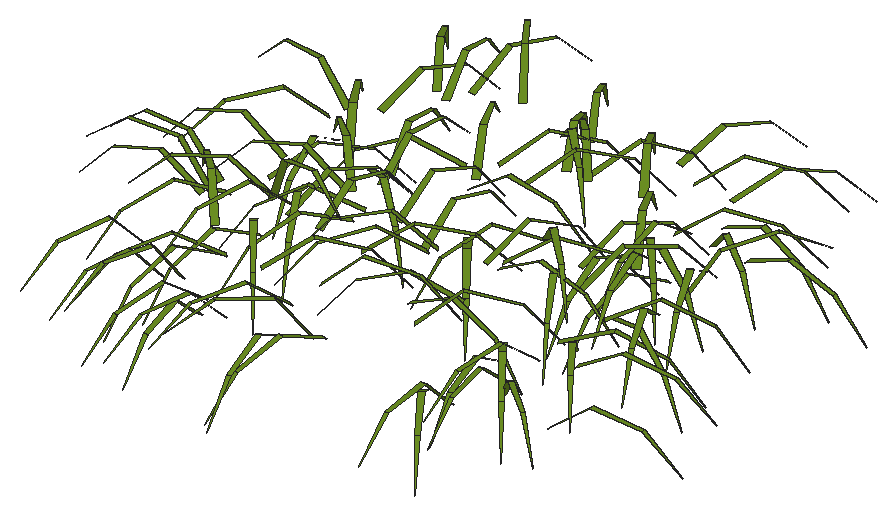
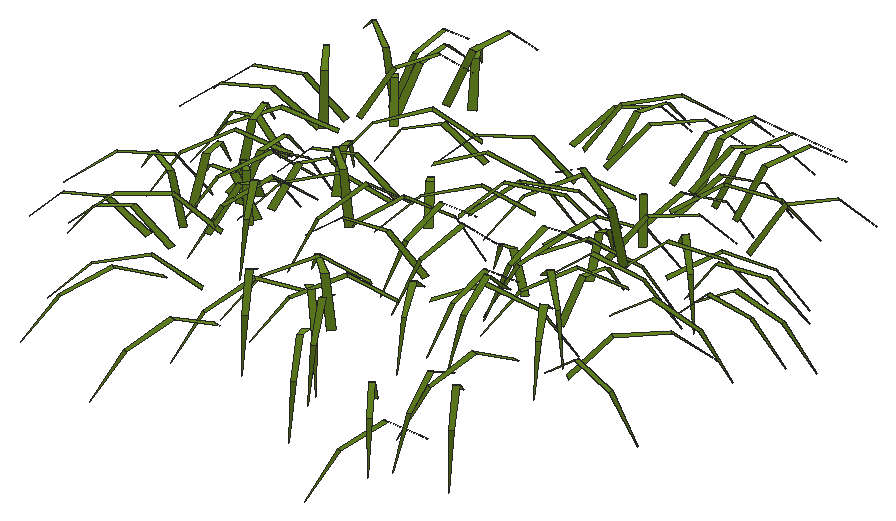
# SketchUp Ruby script. Lengths in inches.
U = 1.inch
M = Sketchup.active_model
def pt(a) = Geom::Point3d.new(a.map { |v| v * U })
def face(e, loops, mat)
  f = e.add_face(loops[0].map { |a| pt(a) })
  loops[1..].each { |l| e.add_face(l.map { |a| pt(a) }).erase! }
  f.material = f.back_material = mat if mat
  f
end
# faces: each face lists its corners as indices into pts; further lists are holes
def faces(e, pts, list, mat = nil) = list.each { |f| face(e, (f[0].is_a?(Array) ? f : [f]).map { |l| l.map { |i| pts[i] } }, mat) }
# xy, xz, yz: faces in a plane at the given z, y or x. An outline is a flat list of corners, or four numbers for a rectangle; further outlines are holes
def ring(l) = l.size == 4 ? [[l[0], l[1]], [l[2], l[1]], [l[2], l[3]], [l[0], l[3]]] : l.each_slice(2).to_a
def flat(e, list, mat, &to3) = list.each { |f| face(e, (f[0].is_a?(Array) ? f : [f]).map { |l| ring(l).map { |u, v| to3.(u, v) } }, mat) }
def xy(e, z, list, mat = nil) = flat(e, list, mat) { |x, y| [x, y, z] }
def xz(e, y, list, mat = nil) = flat(e, list, mat) { |x, z| [x, y, z] }
def yz(e, x, list, mat = nil) = flat(e, list, mat) { |y, z| [x, y, z] }
def lines(e, pts, list) = list.each { |a, b| e.add_line(pt(pts[a]), pt(pts[b])) }
# prism: a flat outline (further loops are holes) pulled along v
def prism(e, loops, v, mat = nil)
  f = face(e, loops, mat); d = Geom::Vector3d.new(v.map { |x| x * U })
  f.pushpull(f.normal.samedirection?(d) ? d.length : -d.length)
end
def box(e, o, s, mat = nil) = prism(e, [[o, [o[0] + s[0], o[1], o[2]], [o[0] + s[0], o[1] + s[1], o[2]], [o[0], o[1] + s[1], o[2]]]], [0, 0, s[2]], mat)
def at(x, y, z, deg = 0) = Geom::Transformation.translation(pt([x, y, z])) * Geom::Transformation.rotation(ORIGIN, Z_AXIS, deg.degrees)
def axes(o, x, y, z) = Geom::Transformation.new([*x, 0, *y, 0, *z, 0, *pt(o).to_a, 1])
def part(name) = M.definitions.add(name)
# library, detail: a bought-in or finely detailed component or shape, given as its bounding box
def library(name, o, s) = part(name).tap { |d| box(d.entities, o, s) }
def detail(e, o, s) = box(e.add_group.entities, o, s)
def put(e, d, t, mat = nil) = e.add_instance(d, t).tap { |i| i.material = mat if mat }
def group(e, t, mat = nil) = e.add_group.tap { |g| g.transformation = t; g.material = mat if mat }.entities
root = M.entities
M.materials.add("[0061_OliveDrab]").color = [107, 142, 35]
p = [[550.53,11.4,559.14],[550.39,11.51,559.14],[549.55,10.29,556.97],[556.85,12.2,559.2],[556.66,12.31,559.2],[556.06,10.94,557.04],
  [577.17,15.06,559.01],[577.09,14.89,559.01],[578.69,14.24,557.03],[571.92,16.4,559.27],[571.73,16.43,559.27],[571.6,15.04,557.05],
  [563.83,16.5,559.26],[563.68,16.61,559.26],[562.95,15.5,556.99],[576.57,16.09,559.07],[576.66,15.91,559.07],[578.05,16.67,556.97],
  [576.4,19.42,559.1875],[576.52,19.23,559.1875],[577.66,20.13,557],[579.22,11.04,558.77],[579.24,10.84,558.77],[581.21,11.15,557.05],
  [578.46,24.97,558.98],[578.45,24.76,558.98],[580.31,24.75,557.13],[572.51,4.17,559.14],[572.34,4.06,559.14],[573.47,2.63,557.24],
  [555.28,6.22,559.4],[555.09,6.27,559.4],[554.83,4.85,557.21],[555.6,8.46,559.36],[555.42,8.51,559.36],[555.14,7.1,557.16],
  [573.62,8.49,559.26],[573.46,8.375,559.26],[574.51,7.18,557.17],[558.04,13.51,559.35],[557.85,13.4,559.35],[558.68,12.14,557.2],
  [566.88,14.53,559.26],[566.7,14.39,559.26],[567.76,13.2,557.17],[554.87,14.97,559.34],[554.78,15.13,559.34],[553.5625,14.3,557.16],
  [555.24,34.98,558.98],[555.45,34.9375,558.98],[555.73,36.81,557.15],[563.09,3.13,559.2],[562.89,3.1,559.2],[563.24,1.35,557.28],
  [563.18,3.54,559.21],[562.98,3.57,559.21],[562.76,1.79,557.3],[558.66,10.34,559.48],[558.5,10.21,559.48],[559.46,9.16,557.26],
  [570.14,12.38,559.46],[570.13,12.17,559.46],[571.64,12.22,557.3125],[560.76,17.37,559.375],[560.62,17.2,559.375],[561.9,16.28,557.27],
  [576.31,25.49,559.35],[576.28,25.28,559.35],[577.93,25.13,557.31],[571.17,14.64,559.53],[571,14.54,559.53],[571.9,13.28,557.41],
  [566.61,30.04,559.53],[566.8,29.93,559.53],[567.41,31.3125,557.38],[574.57,10.62,557.51],[574.61,10.28,557.51],[576.66,10.53,559.12],
  [576.63,10.81,559.12],[547.04,15.13,559.45],[547.03,15.34,559.45],[545.24,15.2,557.54],[559.88,32.26,559.5],[560.05,32.36,559.5],
  [559.0625,33.74,557.48],[567.3,34.4375,559.32],[567.52,34.38,559.32],[567.85,36.24,557.49],[562.55,12.23,559.61],[562.48,12.43,559.61],
  [560.89,11.8,557.61],[555.53,21.01,559.63],[555.44,21.21,559.63],[553.98,20.42,557.59],[560.97,29.51,559.69],[561.16,29.62,559.69],
  [560.25,30.98,557.64],[572.37,32.6,559.48],[572.54,32.52,559.48],[573.27,34.2,557.6],[556.51,3.61,559.64],[556.32,3.66,559.64],
  [555.94,1.98,557.66],[553.4,7.4,559.76],[553.26,7.54,559.76],[552.16,6.32,557.71],[570.82,16.45,559.67],[570.6,16.42,559.67],
  [570.94,14.78,557.65],[551.76,31.6875,559.72],[551.92,31.8,559.72],[550.92,33.11,557.67],[575.17,18.4,559.78],[574.98,18.3125,559.78],
  [575.81,16.75,557.84],[574.3,20.18,559.72],[574.2,19.98,559.72],[575.82,19.26,557.78],[567.33,21.36,560],[567.5,21.29,560],
  [567.95,22.73,557.85],[561.41,28.94,559.77],[561.56,29.07,559.77],[560.34,30.3125,557.8],[578.43,14.28,559.6],[578.46,14.0625,559.6],
  [580.41,14.44,557.89],[555.39,16.89,559.95],[555.2,16.84,559.95],[555.71,15.21,557.95],[564.61,29.63,559.93],[564.79,29.76,559.93],
  [563.74,31.1,557.93],[554.22,30.41,557.93],[554.58,30.33,557.93],[554.97,32.41,559.49],[554.68,32.47,559.49],[553.98,31.83,559.83],
  [554.17,31.89,559.83],[553.56,33.58,557.92],[558.76,2.94,559.78],[558.54,2.91,559.78],[558.97,0.99,558.03],[575.71,14.72,559.85],
  [575.51,14.62,559.85],[576.43,12.99,558.01],[561.77,14.38,559.99],[561.93,14.22,559.99],[563.02,15.55,558],[570.9,19.88,560.08],
  [570.7,19.88,560.08],[570.8,18.24,558.03],[554.7,29.54,559.86],[554.92,29.51,559.86],[555.13,31.3125,557.96],[573.12,19.4375,560.05],
  [572.96,19.3,560.05],[574.16,18.09,558.05],[563.9,27.65,560.14],[564.07,27.5,560.14],[565.08,28.84,558.12],[551.22,6.32,560.12],
  [551.03,6.4,560.12],[550.46,4.66,558.23],[571.4,16.92,560.07],[571.39,16.74,560.07],[573.26,16.72,558.22],[548.57,18.87,560.14],
  [548.56,19.0625,560.14],[546.82,18.92,558.19],[556.6,21.06,560.15],[556.75,20.95,560.15],[557.6875,22.45,558.21],[571.23,3.66,560.02],
  [571.01,3.66,560.02],[571.18,1.7,558.27],[558.22,19.67,560.24],[558.44,19.67,560.24],[558.29,21.46,558.32],[570.3,20.26,560.21],
  [570.4,20.1,560.21],[571.875,21.1875,558.32],[565.86,27.07,560.25],[566.01,26.94,560.25],[567.09,28.31,558.29],[571.19,8.14,558.45],
  [570.81,8.125,558.45],[570.9,6.26,560.3],[571.21,6.27,560.3],[560.04,12.84,560.26],[559.89,12.98,560.26],[558.69,11.6,558.375],
  [557.85,19.62,560.32],[558.05,19.5625,560.32],[558.44,21.29,558.38],[562.86,20.9375,560.33],[563.08,20.9375,560.33],[562.96,22.66,558.35],
  [561.2,22.03,560.45],[561.4,22,560.45],[561.54,23.64,558.39],[570.74,23.59,560.39],[570.93,23.51,560.39],[571.45,25.12,558.375],
  [572.1875,30.72,560.27],[572.29,30.56,560.27],[573.83,31.64,558.43],[554.67,33.61,560.16],[554.83,33.73,560.16],[553.61,35.23,558.375],
  [572.46,6.46,560.1875],[572.25,6.41,560.1875],[572.8125,4.47,558.51],[558.08,7.52,558.49],[557.69,7.46,558.49],[558.07,5.46,560.15],
  [558.375,5.51,560.15],[570.24,14.08,560.42],[570.37,13.91,560.42],[571.65,15.08,558.45],[556.71,24.71,560.51],[556.9,24.76,560.51],
  [556.37,26.39,558.52],[559.22,7.69,558.64],[558.89,7.76,558.64],[558.52,5.93,560.48],[558.78,5.87,560.48],[572.59,9.94,558.64],
  [572.375,9.69,558.64],[573.88,8.46,560.4],[574.05,8.66,560.4],[554.53,11.63,560.52],[554.33,11.71,560.52],[553.76,10.02,558.6],
  [572.58,17.17,560.48],[572.38,17.12,560.48],[572.92,15.33,558.625],[564.8,17.625,560.37],[564.92,17.48,560.37],[566.39,18.76,558.6],
  [549.32,19.99,560.3],[549.13,20.12,560.3],[548.05,18.41,558.63],[553.99,21.69,560.4375],[554.13,21.83,560.4375],[552.7,23.1,558.64],
  [572.31,21.95,560.53],[572.51,21.85,560.53],[573.19,23.48,558.58],[547.98,25.62,560.33],[548.04,25.8,560.33],[546.125,26.28,558.59],
  [557.26,29.98,558.63],[557.54,30.18,558.63],[556.41,31.66,560.48],[556.18,31.49,560.48],[558.18,3.32,560.35],[558,3.36,560.35],
  [557.65,1.32,558.72],[576.03,6.93,560.3],[575.91,6.79,560.3],[577.58,5.5,558.74],[569.79,8.1875,558.67],[569.5,7.98,558.67],
  [570.86,6.09,559.88],[571.1,6.26,559.88],[552.91,10.39,558.6875],[552.58,10.53,558.6875],[551.94,8.82,560.58],[552.21,8.71,560.58],
  [551.45,15.89,560.51],[551.6,16.02,560.51],[550.24,17.32,558.67],[552.69,17.54,560.6],[552.67,17.73,560.6],[550.87,17.37,558.72],
  [559.42,5.09,560.53],[559.23,5.18,560.53],[558.47,3.37,558.78],[562.48,7.93,558.76],[562.13,7.88,558.76],[562.49,5.58,559.98],
  [562.78,5.62,559.98],[571.86,7.67,560.5],[571.68,7.7,560.5],[571.52,5.71,558.8],[555.07,8.66,558.77],[554.74,8.71,558.77],
  [554.52,6.96,560.71],[554.79,6.92,560.71],[573.6,13.7,558.8125],[573.65,13.32,558.8125],[575.91,13.66,560.1],[575.87,13.98,560.1],
  [551.81,15.15,558.78],[551.8,15.51,558.78],[549.5625,15.43,560.15],[549.57,15.14,560.15],[551.75,16.45,558.75],[551.78,16.8,558.75],
  [549.87,16.99,560.54],[549.84,16.7,560.54],[547.24,17.04,560.4],[547.26,17.24,560.4],[545.18,17.37,558.8],[575.95,21.92,560.57],
  [575.83,21.77,560.57],[577.43,20.73,558.75],[552.05,23.69,558.84],[551.74,23.92,558.84],[550.61,22.28,560.55],[550.87,22.09,560.55],
  [564.99,24.59,560.56],[564.83,24.43,560.56],[566.28,23.18,558.76],[573.53,25.37,558.77],[573.51,25,558.77],[575.9375,24.88,559.75],
  [575.96,25.18,559.75],[573.04,5.84,560.46],[572.86,5.8,560.46],[573.34,3.72,558.93],[557.88,8.07,558.89],[557.54,8.17,558.89],
  [556.97,6.09,560.39],[557.25,6.01,560.39],[559.72,14.17,560.75],[559.61,14.34,560.75],[558.15,13.23,558.86],[573.7,18.99,558.92],
  [573.35,18.82,558.92],[574.33,16.9,560.42],[574.62,17.04,560.42],[573.43,20.95,558.89],[573.71,20.74,558.89],[574.62,22.03,560.99],
  [574.38,22.2,560.99],[557.6,24.3125,560.62],[557.81,24.33,560.62],[557.54,26.29,558.89],[568.73,24.39,560.83],[568.92,24.51,560.83],
  [567.9,26,558.92],[552.77,24.51,560.5625],[552.96,24.64,560.5625],[551.74,26.27,558.9],[574.8,25.96,560.625],[574.88,25.78,560.625],
  [576.67,26.63,558.9],[566.07,29.68,558.93],[566.46,29.58,558.93],[566.98,31.91,560.02],[566.67,31.99,560.02],[563.61,8.11,558.98],
  [563.34,8.36,558.98],[562.28,7.11,561.04],[562.5,6.91,561.04],[556.14,8.6875,559.04],[555.82,8.77,559.04],[555.48,7.22,561.13],
  [555.74,7.15,561.13],[572.27,10.45,558.95],[571.96,10.39,558.95],[572.36,8.375,560.59],[572.61,8.42,560.59],[575.99,10.25,560.59],
  [575.8125,10.12,560.59],[577.18,8.51,559.03],[565.77,12.74,560.85],[565.83,12.54,560.85],[567.61,13.19,559.03],[550.92,14.27,560.75],
  [550.85,14.47,560.75],[549.06,13.75,558.97],[575,16.13,560.02],[574.88,15.88,560.02],[552.13,15.29,558.99],[552.11,15.6,558.99],
  [550.57,15.45,561.11],[550.59,15.1875,561.11],[566.02,21.55,560.62],[566.01,21.35,560.62],[568.0625,21.32,558.99],[558.46,26.55,560.63],
  [558.63,26.65,560.63],[557.53,28.375,558.98],[554.39,4.33,560.7],[554.2,4.36,560.7],[554,2.26,559.13],[564.14,8.36,559.09],
  [563.8,8.43,559.09],[563.39,6.02,560.0625],[563.67,5.97,560.0625],[552,13.21,560.34],[551.79,13.375,560.34],[574.4,15.12,560.18],
  [574.53,14.86,560.18],[569.9,17.23,560.82],[569.74,17.07,560.82],[571.23,15.79,559.07],[552.45,24.2,559.125],[552.55,24.52,559.125],
  [550.54,25.09,560.71],[550.46,24.83,560.71],[554.32,27.79,559.14],[554.61,27.99,559.14],[553.35,29.78,560.58],[553.11,29.62,560.58],
  [572.53,12.31,559.24],[572.21,12.35,559.24],[571.97,10.28,560.84],[572.23,10.25,560.84],[557.99,14.24,560.41],[557.72,14.38,560.41],
  [573.21,14.03,559.18],[572.9,13.8,559.18],[574.1875,12.17,560.78],[574.44,12.36,560.78],[574.4375,18.16,560.4],[574.61,17.9,560.4],
  [573.27,22.77,559.1875],[572.94,22.62,559.1875],[573.9,20.58,560.54],[574.18,20.71,560.54],[570.11,28.24,559.2],[570.41,28.09,559.2],
  [571.46,30.25,560.26],[571.21,30.375,560.26],[561.53,9.28,559.35],[561.2,9.44,559.35],[560.32,7.53,560.93],[560.59,7.4,560.93],
  [572.1875,10.4,560.36],[571.97,10.23,560.36],[571.45,11.2,559.27],[571.09,11.11,559.27],[571.63,8.92,560.62],[571.93,8.99,560.62],
  [556.9375,15.59,560.51],[556.67,15.4375,560.51],[572.15,14.1,559.32],[572.3,13.78,559.32],[565.47,16.44,560.36],[565.22,16.25,560.36],
  [556.9,16.13,560.54],[556.77,16.36,560.54],[572.73,17.23,559.28],[572.59,16.93,559.28],[572.33,18.67,560.51],[572.07,18.72,560.51],
  [565.24,18.26,560.6],[565.02,18.43,560.6],[572.4375,16.86,559.3],[572.66,16.53,559.3],[572.73,20.96,559.29],[572.41,21.02,559.29],
  [553.25,18.91,559.35],[553.24,19.25,559.35],[551.09,19.17,560.85],[551.1,18.89,560.85],[572.26,24.66,559.31],[572.07,24.39,559.31],
  [573.71,23.25,561],[573.87,23.47,561],[573.91,25.9,560.33],[573.86,25.6,560.33],[571.53,26.3,559.29],[571.48,25.93,559.29],
  [555.3125,27.19,559.33],[555.65,27.3,559.33],[554.95,29.49,560.58],[554.67,29.41,560.58],[568.14,28.27,559.34],[568.32,27.99,559.34],
  [570.14,29.17,560.82],[569.99,29.4,560.82],[555.9,8.48,560.59],[555.625,8.55,560.59],[556.24,10.69,560.58],[555.99,10.76,560.58],
  [556.5,10.75,559.43],[556.17,10.84,559.43],[570.71,12.37,559.44],[570.4375,12.16,559.44],[554.58,12.4375,559.4375],[554.84,12.67,559.4375],
  [553.39,14.18,561.03],[553.18,13.98,561.03],[553.52,15.12,559.375],[553.27,15.3125,559.375],[558.95,18.92,560.48],[558.75,18.68,560.48],
  [553.77,24.79,559.39],[554.15,24.72,559.39],[554.53,27.02,560.6],[554.21,27.07,560.6],[562.42,28.12,559.39],[562.7,28.3,559.39],
  [561.39,30.32,560.4375],[561.16,30.17,560.4375],[556.85,10.6875,559.46],[556.62,10.93,559.46],[554.98,9.28,560.69],[555.17,9.09,560.69],
  [557.26,12.19,560.7],[557.03,12.01,560.7],[556.9,12.99,559.5],[556.59,13.07,559.5],[558.45,10.97,559.5],[558.73,10.7,559.5],
  [560.26,12.38,560.82],[560.03,12.6,560.82],[566.6,11.27,559.5],[566.83,10.98,559.5],[568.42,12.3,561.12],[568.23,12.53,561.12],
  [561.4,11.49,559.5],[561.51,11.13,559.5],[563.36,11.74,561.26],[563.28,12.02,561.26],[555.84,14.05,559.5],[555.56,13.83,559.5],
  [565.39,12.64,559.5],[565.38,12.28,559.5],[567.77,12.22,560.59],[567.78,12.52,560.59],[567.2,13.67,559.5],[567.09,14.02,559.5],
  [564.8,13.23,560.53],[564.9,12.95,560.53],[556.34,15.86,559.5],[555.98,16,559.5],[555.25,14.09,561.14],[555.53,13.98,561.14],
  [559.18,16.4,559.5],[558.85,16.57,559.5],[560.99,14.69,559.5],[561.1875,14.4375,559.5],[562.92,15.85,560.875],[562.76,16.06,560.875],
  [569.95,16.69,560.62],[569.71,16.54,560.62],[563.41,16.1875,559.5],[563.15,16.44,559.5],[561.63,14.83,560.91],[561.84,14.625,560.91],
  [558.25,14.93,559.5],[558.63,14.94,559.5],[558.55,17.14,560.93],[558.24,17.14,560.93],[556.47,15.14,559.5],[556.81,15.04,559.5],
  [557.375,17.12,561.01],[557.1,17.2,561.01],[555.33,15.68,559.5],[555.23,15.97,559.5],[555.21,16.02,559.5],[553.3,15.34,561.16],
  [553.39,15.06,561.16],[555.26,16.04,559.5],[555.11,15.6875,559.5],[556.13,15.3125,561.89],[556.25,15.6,561.89],[555.79,17.72,559.5],
  [555.47,17.54,559.5],[563.51,16.64,559.5],[563.32,16.92,559.5],[561.73,15.81,561.26],[561.88,15.58,561.26],[558.99,17.33,559.5],
  [558.82,17.61,559.5],[562.82,16.31,559.5],[563.2,16.31,559.5],[563.15,18.42,561.0625],[562.84,18.42,561.0625],[563.99,18.43,559.5],
  [563.68,18.2,559.5],[568.73,18.73,559.5],[568.43,18.54,559.5],[566.56,17.28,559.5],[566.54,16.96,559.5],[568.85,16.85,560.73],
  [568.87,17.11,560.73],[553.84,17.19,559.49],[554.1,17.01,559.49],[555.35,18.86,560.88],[555.13,19.01,560.88],[565.66,17.11,559.5],
  [565.96,17,559.5],[566.6875,19.01,561.02],[566.4375,19.11,561.02],[566.26,17.69,559.5],[566.44,17.42,559.5],[568.3,18.68,560.87],
  [568.15,18.9,560.87],[560.46,17.62,559.5],[560.81,17.57,559.5],[561.07,19.52,561.23],[560.79,19.56,561.23],[570.2,17.89,559.5],
  [570.55,17.72,559.5],[571.42,19.55,561.16],[571.14,19.69,561.16],[557.26,18.14,559.5],[557.21,18.47,559.5],[555.2,18.14,561.16],
  [555.24,17.875,561.16],[557.32,18.3,559.5],[557.5625,18.55,559.5],[555.99,20.06,560.96],[555.79,19.86,560.96],[566.71,20.14,559.5],
  [566.47,20.32,559.5],[566.45,20.33,559.5],[557.09,20.5,559.5],[556.85,20.21,559.5],[566.62,20.48,559.5],[566.36,20.21,559.5],
  [567.84,18.84,561.18],[568.05,19.0625,561.18],[570.22,21.25,559.5],[569.84,21.2,559.5],[570.21,18.85,560.6],[570.52,18.89,560.6],
  [554.3,21.52,559.5],[553.97,21.44,559.5],[554.55,19.24,560.8],[554.82,19.3,560.8],[569.01,19.36,559.5],[569.33,19.24,559.5],
  [570.05,21.16,561.14],[569.79,21.26,561.14],[557.91,19.59,559.5],[558.27,19.62,559.5],[558.0625,21.75,561.02],[557.77,21.73,561.02],
  [571.55,21.75,559.5],[571.2,21.67,559.5],[571.73,19.6,561.03],[572.02,19.67,561.03],[557.79,20.3125,559.5],[558.12,20.4,559.5],
  [557.58,22.32,561.2],[557.3125,22.25,561.2],[555.36,20.47,559.5],[555.68,20.6875,559.5],[554.4375,22.5,560.93],[554.17,22.32,560.93],
  [570.93,20.52,559.5],[571.26,20.72,559.5],[570.27,22.3125,561.34],[570,22.15,561.34],[570,22.49,559.5],[569.82,22.15,559.5],
  [571.97,21.08,560.57],[572.11,21.36,560.57],[570.06,23.05,559.5],[569.79,22.81,559.5],[571.28,21.15,560.875],[571.51,21.34,560.875],
  [561.24,21.91,559.5],[561.22,21.58,559.5],[563.4,21.47,560.95],[563.42,21.75,560.95],[559.96,22.93,559.5],[559.81,23.27,559.5],
  [557.65,22.25,560.59],[557.77,21.97,560.59],[560.78,22.375,559.5],[561.07,22.54,559.5],[559.96,24.42,560.97],[559.72,24.28,560.97],
  [570.99,24.54,559.49],[570.64,24.54,559.49],[570.67,22.36,560.95],[570.95,22.36,560.95],[562.7,23.6,559.5],[562.95,23.38,559.5],
  [564.36,25.03,560.98],[564.16,25.21,560.98],[560.77,24.18,559.5],[561.0625,23.92,559.5],[562.47,25.59,560.96],[562.23,25.8,560.96],
  [570.41,24.2,559.5],[570.54,23.89,559.5],[572.5,24.74,561.03],[572.39,25,561.03],[563.29,25.3125,559.5],[563.63,25.5,559.5],
  [562.42,27.53,560.66],[562.15,27.37,560.66],[564.56,25.25,559.5],[564.8125,25.47,559.5],[563.23,27.23,560.63],[563.02,27.05,560.63],
  [567.24,25.64,559.5],[567.55,25.86,559.5],[566.23,27.73,560.78],[565.97,27.55,560.78],[564.31,25.9,559.5],[564.65,25.72,559.5],
  [565.73,27.82,560.65],[565.45,27.97,560.65],[561.68,27.93,559.48],[561.41,27.65,559.48],[562.95,26.2,561.04],[563.17,26.43,561.04],
  [555.09,4.61,561.19],[554.9,4.66,561.19],[554.51,2.6,559.6],[547.98,15.01,561.21],[547.96,15.1875,561.21],[545.875,14.92,559.63],
  [560.74,4.98,561.23],[560.58,5.12,561.23],[559.22,3.41,559.77],[575.94,24.25,561.52],[576.1,24.125,561.52],[577.42,26.09,560.37],
  [558.58,14.6,562.58],[558.49,14.4,562.58],[560.66,13.63,561.3]]
faces(root,p,[[0,1,2],[3,4,5],[6,7,8],[9,10,11],[12,13,14],[15,16,17],[18,19,20],[21,22,23],
  [24,25,26],[27,28,29],[30,31,32],[33,34,35],[36,37,38],[39,40,41],[42,43,44],[45,46,47],
  [48,49,50],[51,52,53],[54,55,56],[57,58,59],[60,61,62],[63,64,65],[66,67,68],[69,70,71],
  [72,73,74],[75,76,77,78],[79,80,81],[82,83,84],[85,86,87],[88,89,90],[91,92,93],[94,95,96],
  [97,98,99],[100,101,102],[103,104,105],[106,107,108],[109,110,111],[112,113,114],[115,116,117],[118,119,120],
  [121,122,123],[124,125,126],[127,128,129],[130,131,132],[133,134,135,136],[137,138,139],[140,141,142],[143,144,145],
  [146,147,148],[149,150,151],[152,153,154],[155,156,157],[158,159,160],[161,162,163],[164,165,166],[167,168,169],
  [170,171,172],[173,174,175],[176,177,178],[179,180,181],[182,183,184],[185,186,187,188],[189,190,191],[192,193,194],
  [195,196,197],[198,199,200],[201,202,203],[204,205,206],[207,208,209],[210,211,212],[213,214,215,216],[217,218,219],
  [220,221,222],[223,224,225,226],[227,228,229,230],[231,232,233],[234,235,236],[237,238,239],[240,241,242],[243,244,245],
  [246,247,248],[249,250,251],[252,253,254,255],[256,257,258],[259,260,261],[262,263,264,265],[266,267,268,269],[270,271,272],
  [273,274,275],[276,277,278],[279,280,281,282],[283,284,285],[286,287,288,289],[78,77,22,21],[290,291,292,293],[294,295,296,297],
  [298,299,300,301],[302,303,304],[305,306,307],[308,309,310,311],[312,313,314],[315,316,317,318],[319,320,321],[322,323,324,325],
  [326,327,328],[329,330,331,332],[333,334,335,336],[337,338,339],[340,341,342],[343,344,345],[346,347,348],[349,350,351,352],
  [353,354,355,356],[357,358,359,360],[361,362,363,364],[365,366,367],[368,369,370],[371,372,373],[374,375,7,6],[376,377,378,379],
  [380,381,382],[318,317,25,24],[383,384,385],[136,135,49,48],[386,387,388],[265,264,28,27],[389,390,391,392],[393,394,1,0],
  [395,396,16,15],[397,398,399],[400,401,402,403],[404,405,406,407],[282,281,52,51],[392,391,55,54],[408,409,410,411],[412,413,4,3],
  [414,415,416,417],[418,419,19,18],[420,421,422,423],[424,425,426,427],[428,429,430,431],[432,433,37,36],[434,435,436,437],[438,439,40,39],
  [440,441,396,395],[442,443,43,42],[444,445,46,45],[446,447,375,374],[448,449,10,9],[450,451,13,12],[452,453,419,418],[454,455,449,448],
  [456,457,458,459],[460,461,462,463],[464,465,67,66],[466,467,465,464],[468,469,470,471],[472,473,474,475],[352,351,86,85],[476,477,31,30],
  [478,479,34,33],[480,481,477,476],[482,483,433,432],[484,485,486,487],[488,489,394,393],[490,491,64,63],[492,493,494,495],[496,497,498,499],
  [500,501,502,503],[504,505,58,57],[506,507,479,478],[508,509,510,511],[512,513,514,515],[516,517,518,519],[520,521,505,504],[522,523,524,525],
  [525,524,61,60],[526,527,528,529],[530,531,532,533],[534,535,413,412],[536,537,538,539],[540,541,70,69],[542,543,544,545],[546,547,548,549],
  [550,551,552,553],[297,296,80,79],[554,555,556,557,558],[559,555,560,561,562],[563,564,439,438],[565,566,567,568],[569,570,445,444],[571,572,573,574],
  [575,576,443,442],[577,578,541,540],[579,580,581,582],[583,584,585,586],[587,588,589,590],[591,592,593,594],[595,596,597,598],[599,600,601,602],
  [603,604,605,606],[607,608,609,610],[611,612,613,451,450],[614,615,491,490],[616,612,617,618,619],[620,621,622,623],[624,625,626,627],[628,629,630,631],
  [632,633,634,635],[636,637,638,639],[640,641,642,643],[644,645,646,647],[648,649,650,651],[652,653,654,655],[656,657,658,659],[660,661,662,663],
  [664,665,666,667],[668,669,670,671],[672,673,674,675],[676,677,678,679],[680,681,682,683],[684,685,686,687],[688,689,690,691],[692,693,694,695],
  [696,697,698,699],[700,701,702,703],[704,705,706,707],[703,702,73,72],[499,498,83,82],[427,426,98,97],[708,709,710],[325,324,101,100],
  [529,528,89,88],[293,292,125,124],[711,712,713],[667,666,92,91],[623,622,107,106],[655,654,116,115],[691,690,95,94],[407,406,110,109],
  [216,215,141,140],[714,715,716],[503,502,104,103],[423,422,113,112],[695,694,122,121],[471,470,138,137],[332,331,144,143],[495,494,153,152],
  [699,698,131,130],[188,187,174,173],[511,510,147,146],[627,626,128,127],[590,589,119,118],[269,268,162,161],[582,581,165,164],[459,458,168,167],
  [659,658,156,155],[675,674,150,149],[683,682,159,158],[437,436,211,210],[549,548,177,176],[594,593,180,179],[586,585,171,170],[679,678,183,182],
  [255,254,208,207],[226,225,257,256],[230,229,260,259],[545,544,190,189],[553,552,193,192],[574,573,196,195],[311,310,241,240],[403,402,250,249],
  [475,474,205,204],[515,514,218,217],[539,538,238,237],[301,300,303,302],[598,597,199,198],[610,609,244,243],[631,630,202,201],[717,718,719],
  [431,430,277,276],[364,363,320,319],[411,410,284,283],[533,532,232,231],[487,486,271,270],[639,638,235,234],[602,601,247,246],[643,642,221,220],
  [417,416,366,365],[606,605,274,273],[663,662,381,380],[635,634,338,337],[463,462,306,305],[647,646,344,343],[671,670,384,383],[707,706,313,312],
  [687,686,347,346],[289,288,387,386],[568,567,327,326],[558,557,372,371],[519,518,369,368],[619,618,398,397],[651,650,341,340],[356,355,715,714],
  [336,335,718,717],[360,359,709,708],[379,378,712,711],[720,721,722],[562,561,721,720]],"[0061_OliveDrab]")
